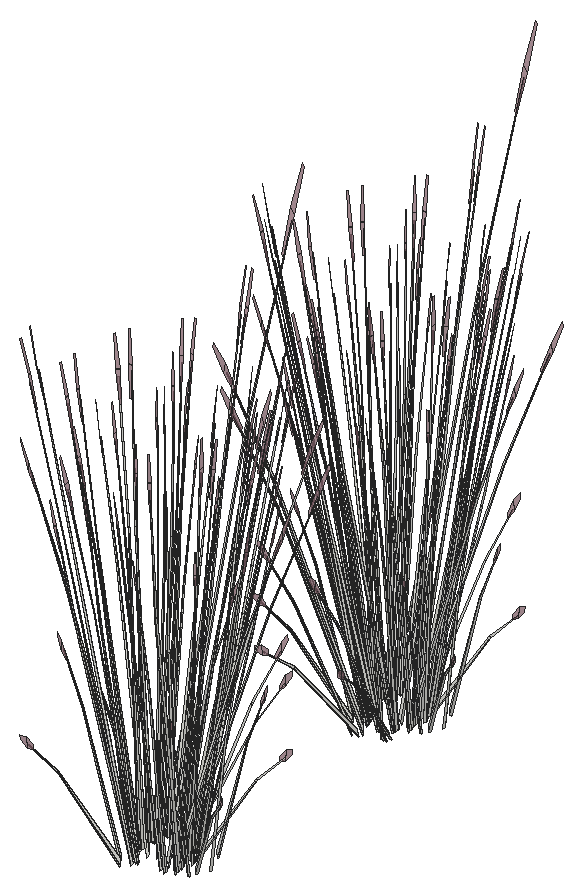
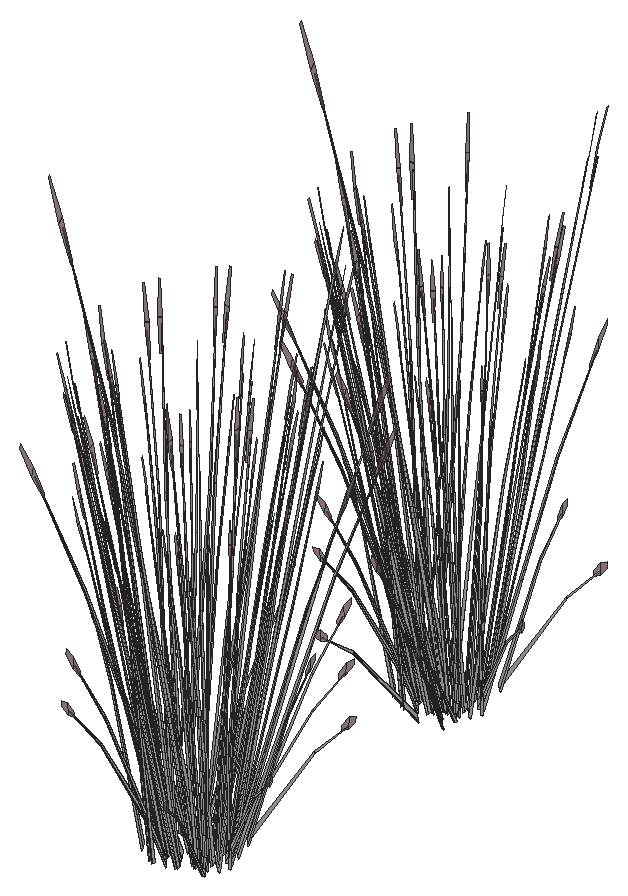
# SketchUp Ruby script. Lengths in inches.
U = 1.inch
M = Sketchup.active_model
def pt(a) = Geom::Point3d.new(a.map { |v| v * U })
def face(e, loops, mat)
  f = e.add_face(loops[0].map { |a| pt(a) })
  loops[1..].each { |l| e.add_face(l.map { |a| pt(a) }).erase! }
  f.material = f.back_material = mat if mat
  f
end
# faces: each face lists its corners as indices into pts; further lists are holes
def faces(e, pts, list, mat = nil) = list.each { |f| face(e, (f[0].is_a?(Array) ? f : [f]).map { |l| l.map { |i| pts[i] } }, mat) }
# xy, xz, yz: faces in a plane at the given z, y or x. An outline is a flat list of corners, or four numbers for a rectangle; further outlines are holes
def ring(l) = l.size == 4 ? [[l[0], l[1]], [l[2], l[1]], [l[2], l[3]], [l[0], l[3]]] : l.each_slice(2).to_a
def flat(e, list, mat, &to3) = list.each { |f| face(e, (f[0].is_a?(Array) ? f : [f]).map { |l| ring(l).map { |u, v| to3.(u, v) } }, mat) }
def xy(e, z, list, mat = nil) = flat(e, list, mat) { |x, y| [x, y, z] }
def xz(e, y, list, mat = nil) = flat(e, list, mat) { |x, z| [x, y, z] }
def yz(e, x, list, mat = nil) = flat(e, list, mat) { |y, z| [x, y, z] }
def lines(e, pts, list) = list.each { |a, b| e.add_line(pt(pts[a]), pt(pts[b])) }
# prism: a flat outline (further loops are holes) pulled along v
def prism(e, loops, v, mat = nil)
  f = face(e, loops, mat); d = Geom::Vector3d.new(v.map { |x| x * U })
  f.pushpull(f.normal.samedirection?(d) ? d.length : -d.length)
end
def box(e, o, s, mat = nil) = prism(e, [[o, [o[0] + s[0], o[1], o[2]], [o[0] + s[0], o[1] + s[1], o[2]], [o[0], o[1] + s[1], o[2]]]], [0, 0, s[2]], mat)
def at(x, y, z, deg = 0) = Geom::Transformation.translation(pt([x, y, z])) * Geom::Transformation.rotation(ORIGIN, Z_AXIS, deg.degrees)
def axes(o, x, y, z) = Geom::Transformation.new([*x, 0, *y, 0, *z, 0, *pt(o).to_a, 1])
def part(name) = M.definitions.add(name)
# library, detail: a bought-in or finely detailed component or shape, given as its bounding box
def library(name, o, s) = part(name).tap { |d| box(d.entities, o, s) }
def detail(e, o, s) = box(e.add_group.entities, o, s)
def put(e, d, t, mat = nil) = e.add_instance(d, t).tap { |i| i.material = mat if mat }
def group(e, t, mat = nil) = e.add_group.tap { |g| g.transformation = t; g.material = mat if mat }.entities
root = M.entities
M.materials.add("LightPink_Translucent").color = [144, 107, 117]
M.materials["LightPink_Translucent"].alpha = 0.75
c1 = part("blade")
p = [[2.15,0.21,22],[0,0.17,0],[0.09,0.45,0],[2.18,0.31,22],[2.29,0.31,22],[0.38,0.45,0],
  [2.48,0.24,33],[2.49,0.24,33],[2.48,0.22,33]]
faces(c1.entities,p,[[0,1,2,3],[4,5,2,3],[6,3,4,7],[8,0,3,6]])
c2 = part("seeds")
p = [[0.3,-0.1,1.38],[-0.01,-0.03,1.59],[-0.01,-0.03,0.03],[0.14,-0.07,-0.07],[0.29,-0.03,3],[0.15,0.01,3.11]]
faces(c2.entities,p,[[0,1,2,3],[1,0,4,5]],"LightPink_Translucent")
c3 = part("blade with seeds")
put(c3.entities,c1,at(0,0,0))
put(c3.entities,c2,axes([2.4,0.25,30.99],[1.5799,-0.05474,1.17369],[-0.12525,1.92788,0.29478],[-0.07173,-0.02425,1.56792]))
put(root,c3,axes([432.04,136.96,2.67],[-0.25113,0.52899,-0.11713],[-0.36369,-0.30476,-0.65011],[-0.12642,-0.14945,0.98783]))
put(root,c3,axes([433.75,137.54,2.07],[0.30922,0.02571,0.0553],[-0.00848,0.38824,0.43534],[0.03236,-0.14872,0.66383]))
put(root,c3,axes([433.52,137.8,2.34],[-0.2546,0.29052,0.30456],[-0.24101,-0.33173,-0.39319],[0.03667,-0.16855,0.75234]))
put(root,c3,axes([431.07,136.81,2.05],[-0.08096,-0.00389,1.50452],[-0.25776,0.38949,-0.23794],[-0.13753,-0.07958,0.12066]))
put(root,c3,axes([434.13,138.74,2.33],[-0.34807,-0.30426,-0.10458],[0.20053,-0.44063,-0.58045],[0.09834,-0.15317,0.88199]))
put(root,c3,axes([432.01,137.4,2.34],[0.05812,0.44446,0.30456],[-0.33222,0.11736,-0.39319],[-0.08923,-0.12737,0.75234]))
put(root,c3,axes([431.01,137.6875,2.38],[0.31075,-0.40722,0.46236],[0.268,0.43246,0.38124],[-0.14579,-0.07512,0.95674]))
put(root,c3,axes([434.99,138.61,2.05],[-0.04915,-0.00419,1.5255],[-0.20409,-0.44904,-0.14414],[0.08196,-0.14765,0.26996]))
put(root,c3,axes([431.16,137.68,2.07],[0.01895,-0.4196,0.0553],[0.28611,0.0115,0.43534],[-0.1096,-0.04391,0.66383]))
put(root,c3,axes([433.96,138.7,2.34],[-0.32754,0.07886,0.30456],[-0.08649,-0.45081,-0.39319],[0.09386,-0.12109,0.75234]))
put(root,c3,axes([434.26,138.63,2.07],[0.25832,0.23207,0.0553],[-0.1504,0.33047,0.43534],[0.08282,-0.10684,0.66383]))
put(root,c3,axes([434.1875,138.53,2.07],[0.09332,0.50785,0.41282],[-0.36608,0.08814,0.34039],[0.10789,-0.11944,0.85423]))
put(root,c3,axes([435.17,139.15,2.05],[0.05222,-0.08405,1.50452],[-0.06683,-0.51557,-0.23794],[0.13101,-0.09775,0.12066]))
put(root,c3,axes([430.76,137.14,2.05],[0.0279,0.05507,1.5255],[-0.13448,0.49501,-0.14414],[-0.1362,0.00358,0.26996]))
put(root,c3,axes([431.35,138,2.34],[0.2141,0.34548,0.30456],[-0.24447,0.32704,-0.39319],[-0.12421,-0.04976,0.75234]))
put(root,c3,axes([431.29,137.78,2.33],[-0.02015,0.56117,-0.10458],[-0.38148,-0.01534,-0.58045],[-0.14692,-0.03898,0.88199]))
put(root,c3,axes([434.15,139.93,2.33],[-0.18933,-0.49965,-0.10458],[0.33602,-0.24554,-0.58045],[0.1416,-0.06592,0.88199]))
put(root,c3,axes([430.81,138.55,1.33],[0.15608,-0.0125,1.47384],[-0.10354,0.54165,0.11917],[-0.22242,-0.0335,0.63005]))
put(root,c3,axes([434.01,139.78,2.34],[-0.31272,-0.15393,0.30456],[0.09121,-0.44909,-0.39319],[0.1259,-0.04118,0.75234]))
put(root,c3,axes([430.74,138.96,2.07],[0.10631,-0.50312,0.41282],[0.34951,0.17204,0.34039],[-0.13745,0.03024,0.85423]))
put(root,c3,axes([430.71,138.83,2.07],[-0.1382,-0.37624,0.0553],[0.25202,-0.18416,0.43534],[-0.11109,0.03633,0.66383]))
put(root,c3,axes([433.49,139.18,1.33],[-0.15608,0.0125,1.47384],[0.10354,-0.54165,0.11917],[0.22242,0.0335,0.63005]))
put(root,c3,axes([434.3,139.92,2.07],[0.1382,0.37624,0.0553],[-0.25202,0.18416,0.43534],[0.11109,-0.03633,0.66383]))
put(root,c3,axes([434.27,139.79,2.07],[-0.10631,0.50312,0.41282],[-0.34951,-0.17204,0.34039],[0.13745,-0.03024,0.85423]))
put(root,c3,axes([431,138.97,2.34],[0.31272,0.15393,0.30456],[-0.09121,0.44909,-0.39319],[-0.1259,0.04118,0.75234]))
put(root,c3,axes([434.9,141.42,2.05],[-0.03403,-0.04831,1.5255],[0.07443,-0.51782,-0.14414],[0.13402,-0.03308,0.26996]))
put(root,c3,axes([430.47,139.31,2.05],[-0.06145,0.07164,1.50452],[0.00523,0.52344,-0.23794],[-0.14085,0.06807,0.12066]))
put(root,c3,axes([430.87,138.82,2.33],[0.18933,0.49965,-0.10458],[-0.33602,0.24554,-0.58045],[-0.1416,0.06592,0.88199]))
put(root,c3,axes([434.6,140.98,1.38],[-0.07202,-0.46385,-0.03003],[0.3404,-0.10664,-0.13615],[0.07108,0.02941,0.44908]))
put(root,c3,axes([433.72,140.97,2.33],[0.02015,-0.56117,-0.10458],[0.38148,0.01534,-0.58045],[0.14692,0.03898,0.88199]))
put(root,c3,axes([433.66,140.75,2.34],[-0.2141,-0.34548,0.30456],[0.24447,-0.32704,-0.39319],[0.12421,0.04976,0.75234]))
put(root,c3,axes([434.05,140.63,2.05],[0.08072,-0.00933,1.50452],[0.22141,-0.42869,-0.23794],[0.14358,0.05659,0.12066]))
put(root,c3,axes([430.82,140.21,2.07],[-0.09332,-0.50785,0.41282],[0.36608,-0.08814,0.34039],[-0.10789,0.11944,0.85423]))
put(root,c3,axes([430.75,140.12,2.07],[-0.25832,-0.23207,0.0553],[0.1504,-0.33047,0.43534],[-0.08282,0.10684,0.66383]))
put(root,c3,axes([430.87,139.5,1.33],[0.13056,-0.11672,1.47384],[0.10992,0.53933,0.11917],[-0.20497,0.12189,0.63005]))
put(root,c3,axes([431.05,140.04,2.34],[0.32754,-0.07886,0.30456],[0.08649,0.45081,-0.39319],[-0.09386,0.12109,0.75234]))
put(root,c3,axes([429.79,139.84,2.05],[0.04802,0.0148,1.5255],[0.14856,0.48754,-0.14414],[-0.0983,0.12796,0.26996]))
put(root,c3,axes([433.86,141.0625,2.07],[-0.01895,0.4196,0.0553],[-0.28611,-0.0115,0.43534],[0.1096,0.04391,0.66383]))
put(root,c3,axes([433.88,140.93,2.07],[-0.27746,0.36359,0.41282],[-0.23929,-0.38612,0.34039],[0.13017,0.06707,0.85423]))
put(root,c3,axes([430.31,141.32,2.86],[0.33205,0.14729,-0.05579],[-0.10214,0.45334,-0.25298],[-0.05431,0.06883,0.83441]))
put(root,c3,axes([433,141.35,2.34],[-0.05812,-0.44446,0.30456],[0.33222,-0.11736,-0.39319],[0.08923,0.12737,0.75234]))
put(root,c3,axes([433.2,140.04,1.33],[-0.13977,-0.09507,1.47384],[0.28925,-0.39884,0.11917],[0.18028,0.17992,0.63005]))
put(root,c3,axes([433.22,138.79,1.85],[-0.32515,-0.2867,1.18923],[0.34333,-0.44639,0.51312],[0.10491,0.26901,1.1495]))
put(root,c3,axes([430.88,140,2.33],[0.34807,0.30426,-0.10458],[-0.20053,0.44063,-0.58045],[-0.09834,0.15317,0.88199]))
put(root,c3,axes([432.97,141.58,2.33],[0.22423,-0.47232,-0.10458],[0.32472,0.27211,-0.58045],[0.11288,0.13344,0.88199]))
put(root,c3,axes([431.35,139.87,1.33],[0.09398,-0.16955,1.47384],[0.23731,0.45764,0.11917],[-0.16276,0.20841,0.63005]))
put(root,c3,axes([431.49,140.94,2.34],[0.2546,-0.29052,0.30456],[0.24101,0.33173,-0.39319],[-0.03667,0.16855,0.75234]))
put(root,c3,axes([432.68,141.97,2.05],[0.00111,-0.06681,1.5255],[0.32247,-0.29474,-0.14414],[0.11201,0.1052,0.26996]))
put(root,c3,axes([431.26,141.21,2.07],[-0.30922,-0.02571,0.0553],[0.00848,-0.38824,0.43534],[-0.03236,0.14872,0.66383]))
put(root,c3,axes([431.36,141.24,2.07],[-0.26795,-0.37649,0.41282],[0.28456,-0.3247,0.34039],[-0.04943,0.17664,0.85423]))
put(root,c3,axes([432.21,141.42,2.34],[0.11344,-0.42434,0.30456],[0.33096,0.12377,-0.39319],[0.03035,0.17085,0.75234]))
put(root,c3,axes([433.05,141.75,2.07],[-0.17102,0.35053,0.0553],[-0.24354,-0.20408,0.43534],[0.07874,0.11238,0.66383]))
put(root,c3,axes([432.65,142.93,2.86],[0.26003,-0.31656,-0.05579],[0.23826,0.3467,-0.25298],[0.01677,0.09824,0.83441]))
put(root,c3,axes([433.125,141.65,2.07],[-0.37426,0.12663,0.41282],[-0.06495,-0.49674,0.34039],[0.08802,0.1464,0.85423]))
put(root,c3,axes([431.28,140.29,1.33],[0.07006,-0.18966,1.47384],[0.29392,0.3925,0.11917],[-0.13259,0.24463,0.63005]))
put(root,c3,axes([432.1,141.81,2.07],[-0.27727,0.18753,0.0553],[-0.13571,-0.34197,0.43534],[0.02678,0.15075,0.66383]))
put(root,c3,axes([430.48,141.27,2.05],[-0.00935,0.1092,1.50452],[0.26544,0.37987,-0.23794],[-0.06949,0.17964,0.12066]))
put(root,c3,axes([431.33,141.02,2.64],[0.41355,0.02734,-0.11608],[-0.0113,0.51765,-0.6443],[-0.02873,0.19937,0.97901]))
put(root,c3,axes([432.09,141.6,2.33],[0.36822,-0.25691,-0.10458],[0.18095,0.45596,-0.58045],[0.04858,0.19215,0.88199]))
put(root,c3,axes([432.2,141.77,2.35],[-0.37078,-0.14426,0.45823],[0.12679,-0.47426,0.37783],[0.02228,0.18651,0.9482]))
put(root,c3,axes([432.62,140.6,1.33],[-0.08601,-0.17716,1.47384],[0.39746,-0.14915,0.11917],[0.08983,0.27813,0.63005]))
put(root,c3,axes([430.45,142.39,2.05],[0.04269,-0.03331,1.5255],[0.35284,0.2216,-0.14414],[-0.00829,0.1845,0.26996]))
put(root,c3,axes([431.92,140.6875,1.33],[-0.00921,-0.21179,1.47384],[0.39917,0.1405,0.11917],[-0.02469,0.30182,0.63005]))
put(root,c3,axes([432.01,142.62,2.05],[0.0477,0.08886,1.50452],[0.38493,0.03491,-0.23794],[0.03871,0.19596,0.12066]))
put(root,c3,axes([431.68,158.98,1.33],[0.08601,0.17716,1.47384],[-0.39746,0.14915,0.11917],[-0.08983,-0.27813,0.63005]))
put(root,c3,axes([432.33,157.81,2.05],[-0.05755,-0.07737,1.50452],[-0.38409,0.04905,-0.23794],[-0.0613,-0.18505,0.12066]))
put(root,c3,axes([434.06,158.75,2.05],[-0.00363,-0.10982,1.50452],[-0.30678,-0.3174,-0.23794],[0.04743,-0.1924,0.12066]))
put(root,c3,axes([433.02,159.29,1.33],[-0.07006,0.18966,1.47384],[-0.29392,-0.3925,0.11917],[0.13259,-0.24463,0.63005]))
put(root,c3,axes([433.98,158.36,2.05],[-0.03821,0.04215,1.5255],[-0.37441,-0.1422,-0.14414],[-0.01355,-0.18393,0.26996]))
put(root,c3,axes([431.9375,157.55,2.05],[-0.00702,0.06614,1.5255],[-0.34622,0.24004,-0.14414],[-0.10188,-0.1227,0.26996]))
put(root,c3,axes([431.86,158.73,2.38],[0.41917,-0.14183,0.46236],[0.07275,0.55635,0.38124],[-0.09858,-0.16397,0.95674]))
put(root,c3,axes([432.81,158.83,2.07],[0.37078,0.14426,0.41282],[-0.12679,0.47426,0.34039],[-0.02228,-0.18651,0.85423]))
put(root,c3,axes([432.92,159,2.33],[-0.36822,0.25691,-0.10458],[-0.18095,-0.45596,-0.58045],[-0.04858,-0.19215,0.88199]))
put(root,c3,axes([433.68,159.58,2.33],[-0.41355,-0.02734,-0.10458],[0.0113,-0.51765,-0.58045],[0.02873,-0.19937,0.88199]))
put(root,c3,axes([432.91,158.79,2.07],[0.27727,-0.18753,0.0553],[0.13571,0.34197,0.43534],[-0.02678,-0.15075,0.66383]))
put(root,c3,axes([431.96,158.85,2.07],[0.17102,-0.35053,0.0553],[0.24354,0.20408,0.43534],[-0.07874,-0.11238,0.66383]))
put(root,c3,axes([431.1,159.53,1.33],[0.13977,0.09507,1.47384],[-0.28925,0.39884,0.11917],[-0.18028,-0.17992,0.63005]))
put(root,c3,axes([432.81,159.18,2.34],[-0.11344,0.42434,0.30456],[-0.33096,-0.12377,-0.39319],[-0.03035,-0.17085,0.75234]))
put(root,c3,axes([433.65,159.36,2.07],[0.26795,0.37649,0.41282],[-0.28456,0.3247,0.34039],[0.04943,-0.17664,0.85423]))
put(root,c3,axes([432.04,158.81,2.67],[-0.25113,0.52899,-0.11713],[-0.36369,-0.30476,-0.65011],[-0.12642,-0.14945,0.98783]))
put(root,c3,axes([433.75,159.39,2.07],[0.30922,0.02571,0.0553],[-0.00848,0.38824,0.43534],[0.03236,-0.14872,0.66383]))
put(root,c3,axes([433.52,159.66,2.34],[-0.2546,0.29052,0.30456],[-0.24101,-0.33173,-0.39319],[0.03667,-0.16855,0.75234]))
put(root,c3,axes([431.07,158.66,2.05],[-0.08096,-0.00389,1.50452],[-0.25776,0.38949,-0.23794],[-0.13753,-0.07958,0.12066]))
put(root,c3,axes([434.13,160.59,2.33],[-0.34807,-0.30426,-0.10458],[0.20053,-0.44063,-0.58045],[0.09834,-0.15317,0.88199]))
put(root,c3,axes([432.01,159.25,2.34],[0.05812,0.44446,0.30456],[-0.33222,0.11736,-0.39319],[-0.08923,-0.12737,0.75234]))
put(root,c3,axes([431.01,159.54,2.38],[0.31075,-0.40722,0.46236],[0.268,0.43246,0.38124],[-0.14579,-0.07512,0.95674]))
put(root,c3,axes([434.99,160.46,2.05],[-0.04915,-0.00419,1.5255],[-0.20409,-0.44904,-0.14414],[0.08196,-0.14765,0.26996]))
put(root,c3,axes([431.16,159.54,2.07],[0.01895,-0.4196,0.0553],[0.28611,0.0115,0.43534],[-0.1096,-0.04391,0.66383]))
put(root,c3,axes([433.96,160.55,2.34],[-0.32754,0.07886,0.30456],[-0.08649,-0.45081,-0.39319],[0.09386,-0.12109,0.75234]))
put(root,c3,axes([434.26,160.48,2.07],[0.25832,0.23207,0.0553],[-0.1504,0.33047,0.43534],[0.08282,-0.10684,0.66383]))
put(root,c3,axes([434.1875,160.38,2.07],[0.09332,0.50785,0.41282],[-0.36608,0.08814,0.34039],[0.10789,-0.11944,0.85423]))
put(root,c3,axes([435.17,161,2.05],[0.05222,-0.08405,1.50452],[-0.06683,-0.51557,-0.23794],[0.13101,-0.09775,0.12066]))
put(root,c3,axes([430.76,158.99,2.05],[0.0279,0.05507,1.5255],[-0.13448,0.49501,-0.14414],[-0.1362,0.00358,0.26996]))
put(root,c3,axes([431.35,159.85,2.34],[0.2141,0.34548,0.30456],[-0.24447,0.32704,-0.39319],[-0.12421,-0.04976,0.75234]))
put(root,c3,axes([431.29,159.63,2.33],[-0.02015,0.56117,-0.10458],[-0.38148,-0.01534,-0.58045],[-0.14692,-0.03898,0.88199]))
put(root,c3,axes([434.15,161.78,2.33],[-0.18933,-0.49965,-0.10458],[0.33602,-0.24554,-0.58045],[0.1416,-0.06592,0.88199]))
put(root,c3,axes([430.81,160.4,1.33],[0.15608,-0.0125,1.47384],[-0.10354,0.54165,0.11917],[-0.22242,-0.0335,0.63005]))
put(root,c3,axes([434.01,161.63,2.34],[-0.31272,-0.15393,0.30456],[0.09121,-0.44909,-0.39319],[0.1259,-0.04118,0.75234]))
put(root,c3,axes([430.74,160.8125,2.07],[0.10631,-0.50312,0.41282],[0.34951,0.17204,0.34039],[-0.13745,0.03024,0.85423]))
put(root,c3,axes([430.71,160.68,2.07],[-0.1382,-0.37624,0.0553],[0.25202,-0.18416,0.43534],[-0.11109,0.03633,0.66383]))
put(root,c3,axes([433.49,161.03,1.33],[-0.15608,0.0125,1.47384],[0.10354,-0.54165,0.11917],[0.22242,0.0335,0.63005]))
put(root,c3,axes([434.3,161.77,2.07],[0.1382,0.37624,0.0553],[-0.25202,0.18416,0.43534],[0.11109,-0.03633,0.66383]))
put(root,c3,axes([434.27,161.64,2.07],[-0.10631,0.50312,0.41282],[-0.34951,-0.17204,0.34039],[0.13745,-0.03024,0.85423]))
put(root,c3,axes([431,160.82,2.34],[0.31272,0.15393,0.30456],[-0.09121,0.44909,-0.39319],[-0.1259,0.04118,0.75234]))
put(root,c3,axes([434.9,163.27,2.05],[-0.03403,-0.04831,1.5255],[0.07443,-0.51782,-0.14414],[0.13402,-0.03308,0.26996]))
put(root,c3,axes([430.47,161.17,2.05],[-0.06145,0.07164,1.50452],[0.00523,0.52344,-0.23794],[-0.14085,0.06807,0.12066]))
put(root,c3,axes([430.87,160.67,2.33],[0.18933,0.49965,-0.10458],[-0.33602,0.24554,-0.58045],[-0.1416,0.06592,0.88199]))
put(root,c3,axes([434.6,162.83,1.38],[-0.07202,-0.46385,-0.03003],[0.3404,-0.10664,-0.13615],[0.07108,0.02941,0.44908]))
put(root,c3,axes([433.72,162.82,2.33],[0.02015,-0.56117,-0.10458],[0.38148,0.01534,-0.58045],[0.14692,0.03898,0.88199]))
put(root,c3,axes([433.66,162.6,2.34],[-0.2141,-0.34548,0.30456],[0.24447,-0.32704,-0.39319],[0.12421,0.04976,0.75234]))
put(root,c3,axes([434.05,162.48,2.05],[0.08072,-0.00933,1.50452],[0.22141,-0.42869,-0.23794],[0.14358,0.05659,0.12066]))
put(root,c3,axes([430.82,162.0625,2.07],[-0.09332,-0.50785,0.41282],[0.36608,-0.08814,0.34039],[-0.10789,0.11944,0.85423]))
put(root,c3,axes([430.75,161.97,2.07],[-0.25832,-0.23207,0.0553],[0.1504,-0.33047,0.43534],[-0.08282,0.10684,0.66383]))
put(root,c3,axes([430.87,161.35,1.33],[0.13056,-0.11672,1.47384],[0.10992,0.53933,0.11917],[-0.20497,0.12189,0.63005]))
put(root,c3,axes([431.05,161.9,2.34],[0.32754,-0.07886,0.30456],[0.08649,0.45081,-0.39319],[-0.09386,0.12109,0.75234]))
put(root,c3,axes([429.79,161.69,2.05],[0.04802,0.0148,1.5255],[0.14856,0.48754,-0.14414],[-0.0983,0.12796,0.26996]))
put(root,c3,axes([433.86,162.91,2.07],[-0.01895,0.4196,0.0553],[-0.28611,-0.0115,0.43534],[0.1096,0.04391,0.66383]))
put(root,c3,axes([433.88,162.78,2.07],[-0.27746,0.36359,0.41282],[-0.23929,-0.38612,0.34039],[0.13017,0.06707,0.85423]))
put(root,c3,axes([430.31,163.18,2.86],[0.33205,0.14729,-0.05579],[-0.10214,0.45334,-0.25298],[-0.05431,0.06883,0.83441]))
put(root,c3,axes([433,163.2,2.34],[-0.05812,-0.44446,0.30456],[0.33222,-0.11736,-0.39319],[0.08923,0.12737,0.75234]))
put(root,c3,axes([433.2,161.9,1.33],[-0.13977,-0.09507,1.47384],[0.28925,-0.39884,0.11917],[0.18028,0.17992,0.63005]))
put(root,c3,axes([433.22,160.64,1.85],[-0.32515,-0.2867,1.18923],[0.34333,-0.44639,0.51312],[0.10491,0.26901,1.1495]))
put(root,c3,axes([430.88,161.85,2.33],[0.34807,0.30426,-0.10458],[-0.20053,0.44063,-0.58045],[-0.09834,0.15317,0.88199]))
put(root,c3,axes([432.97,163.43,2.33],[0.22423,-0.47232,-0.10458],[0.32472,0.27211,-0.58045],[0.11288,0.13344,0.88199]))
put(root,c3,axes([431.35,161.72,1.33],[0.09398,-0.16955,1.47384],[0.23731,0.45764,0.11917],[-0.16276,0.20841,0.63005]))
put(root,c3,axes([431.49,162.79,2.34],[0.2546,-0.29052,0.30456],[0.24101,0.33173,-0.39319],[-0.03667,0.16855,0.75234]))
put(root,c3,axes([432.68,163.82,2.05],[0.00111,-0.06681,1.5255],[0.32247,-0.29474,-0.14414],[0.11201,0.1052,0.26996]))
put(root,c3,axes([431.26,163.06,2.07],[-0.30922,-0.02571,0.0553],[0.00848,-0.38824,0.43534],[-0.03236,0.14872,0.66383]))
put(root,c3,axes([431.36,163.09,2.07],[-0.26795,-0.37649,0.41282],[0.28456,-0.3247,0.34039],[-0.04943,0.17664,0.85423]))
put(root,c3,axes([432.21,163.27,2.34],[0.11344,-0.42434,0.30456],[0.33096,0.12377,-0.39319],[0.03035,0.17085,0.75234]))
put(root,c3,axes([433.05,163.6,2.07],[-0.17102,0.35053,0.0553],[-0.24354,-0.20408,0.43534],[0.07874,0.11238,0.66383]))
put(root,c3,axes([432.65,164.79,2.86],[0.26003,-0.31656,-0.05579],[0.23826,0.3467,-0.25298],[0.01677,0.09824,0.83441]))
put(root,c3,axes([433.125,163.51,2.07],[-0.37426,0.12663,0.41282],[-0.06495,-0.49674,0.34039],[0.08802,0.1464,0.85423]))
put(root,c3,axes([431.28,162.14,1.33],[0.07006,-0.18966,1.47384],[0.29392,0.3925,0.11917],[-0.13259,0.24463,0.63005]))
put(root,c3,axes([432.1,163.66,2.07],[-0.27727,0.18753,0.0553],[-0.13571,-0.34197,0.43534],[0.02678,0.15075,0.66383]))
put(root,c3,axes([430.48,163.12,2.05],[-0.00935,0.1092,1.50452],[0.26544,0.37987,-0.23794],[-0.06949,0.17964,0.12066]))
put(root,c3,axes([431.33,162.87,2.64],[0.41355,0.02734,-0.11608],[-0.0113,0.51765,-0.6443],[-0.02873,0.19937,0.97901]))
put(root,c3,axes([432.09,163.45,2.33],[0.36822,-0.25691,-0.10458],[0.18095,0.45596,-0.58045],[0.04858,0.19215,0.88199]))
put(root,c3,axes([432.2,163.62,2.35],[-0.37078,-0.14426,0.45823],[0.12679,-0.47426,0.37783],[0.02228,0.18651,0.9482]))
